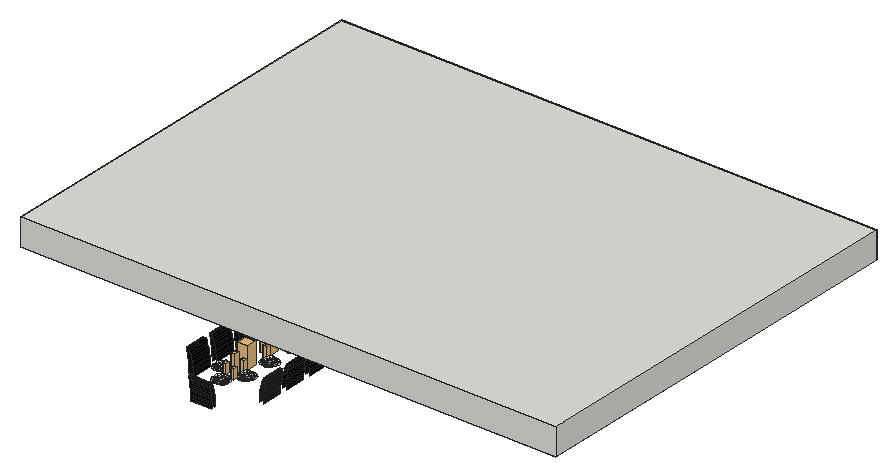
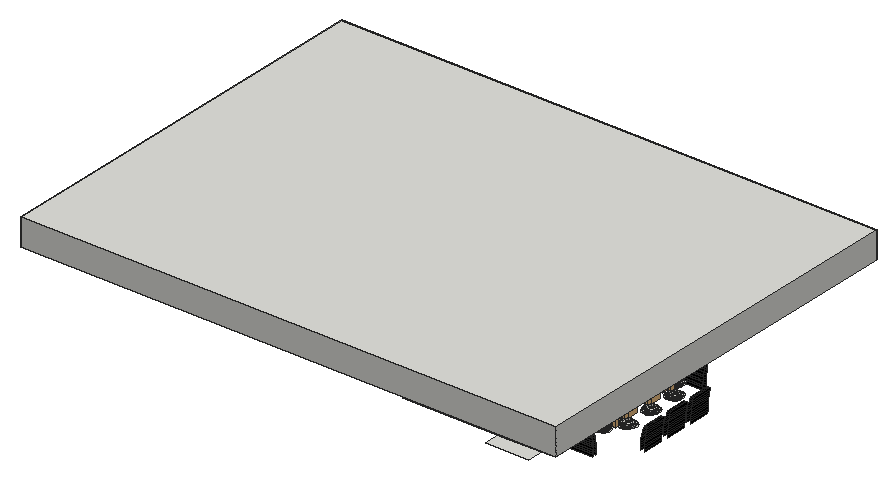
# SketchUp Ruby script. Lengths in inches.
U = 1.inch
M = Sketchup.active_model
def pt(a) = Geom::Point3d.new(a.map { |v| v * U })
def face(e, loops, mat)
  f = e.add_face(loops[0].map { |a| pt(a) })
  loops[1..].each { |l| e.add_face(l.map { |a| pt(a) }).erase! }
  f.material = f.back_material = mat if mat
  f
end
# faces: each face lists its corners as indices into pts; further lists are holes
def faces(e, pts, list, mat = nil) = list.each { |f| face(e, (f[0].is_a?(Array) ? f : [f]).map { |l| l.map { |i| pts[i] } }, mat) }
# xy, xz, yz: faces in a plane at the given z, y or x. An outline is a flat list of corners, or four numbers for a rectangle; further outlines are holes
def ring(l) = l.size == 4 ? [[l[0], l[1]], [l[2], l[1]], [l[2], l[3]], [l[0], l[3]]] : l.each_slice(2).to_a
def flat(e, list, mat, &to3) = list.each { |f| face(e, (f[0].is_a?(Array) ? f : [f]).map { |l| ring(l).map { |u, v| to3.(u, v) } }, mat) }
def xy(e, z, list, mat = nil) = flat(e, list, mat) { |x, y| [x, y, z] }
def xz(e, y, list, mat = nil) = flat(e, list, mat) { |x, z| [x, y, z] }
def yz(e, x, list, mat = nil) = flat(e, list, mat) { |y, z| [x, y, z] }
def lines(e, pts, list) = list.each { |a, b| e.add_line(pt(pts[a]), pt(pts[b])) }
# prism: a flat outline (further loops are holes) pulled along v
def prism(e, loops, v, mat = nil)
  f = face(e, loops, mat); d = Geom::Vector3d.new(v.map { |x| x * U })
  f.pushpull(f.normal.samedirection?(d) ? d.length : -d.length)
end
def box(e, o, s, mat = nil) = prism(e, [[o, [o[0] + s[0], o[1], o[2]], [o[0] + s[0], o[1] + s[1], o[2]], [o[0], o[1] + s[1], o[2]]]], [0, 0, s[2]], mat)
def at(x, y, z, deg = 0) = Geom::Transformation.translation(pt([x, y, z])) * Geom::Transformation.rotation(ORIGIN, Z_AXIS, deg.degrees)
def axes(o, x, y, z) = Geom::Transformation.new([*x, 0, *y, 0, *z, 0, *pt(o).to_a, 1])
def part(name) = M.definitions.add(name)
# library, detail: a bought-in or finely detailed component or shape, given as its bounding box
def library(name, o, s) = part(name).tap { |d| box(d.entities, o, s) }
def detail(e, o, s) = box(e.add_group.entities, o, s)
def put(e, d, t, mat = nil) = e.add_instance(d, t).tap { |i| i.material = mat if mat }
def group(e, t, mat = nil) = e.add_group.tap { |g| g.transformation = t; g.material = mat if mat }.entities
root = M.entities
M.materials.add("[Color M08]").color = [30, 30, 30]
M.materials.add("[Color M09]").color = [0, 0, 0]
c1 = library("Vase with flowers",[0,-0.1,-0.41],[9.125,9.13,19.39])
c2 = library("Candlestick with candle",[0,0,0],[3.93,3.74,15.76])
c3 = library("ske3",[12.02,0,0.58],[3.05,3.06,6.89])
c4 = part("Dishes_Bowl_5in\#1")
xy(c4.entities,0.125,[[-0.25,-0.91,-0.67,-0.67,-0.91,-0.25,-0.91,0.25,-0.67,0.67,-0.25,0.91,0.25,0.91,0.67,0.67,0.91,0.25,0.91,-0.25,0.67,-0.67,0.25,-0.91]])
p = [[-1.16,-1.16,0.41],[-0.67,-0.67,0.125],[-0.25,-0.91,0.125],[-0.43,-1.59,0.41],[0.25,-0.91,0.125],[0.43,-1.59,0.41],
  [0.67,-0.67,0.125],[1.16,-1.16,0.41],[-1.59,-0.43,0.41],[-0.91,-0.25,0.125],[0.91,-0.25,0.125],[1.59,-0.43,0.41],
  [-1.59,0.43,0.41],[-0.91,0.25,0.125],[1.59,0.43,0.41],[0.91,0.25,0.125],[-1.16,1.16,0.41],[-0.67,0.67,0.125],
  [0.67,0.67,0.125],[1.16,1.16,0.41],[-0.43,1.59,0.41],[-0.25,0.91,0.125],[0.25,0.91,0.125],[0.43,1.59,0.41],
  [-1.55,-1.55,0.9375],[-0.57,-2.11,0.9375],[0.57,-2.11,0.9375],[1.55,-1.55,0.9375],[-2.11,-0.57,0.9375],[2.11,-0.57,0.9375],
  [-2.11,0.57,0.9375],[2.11,0.57,0.9375],[-1.55,1.55,0.9375],[1.55,1.55,0.9375],[-0.57,2.11,0.9375],[0.57,2.11,0.9375],
  [-1.77,-1.77,1.625],[-0.65,-2.41,1.625],[0.65,-2.41,1.625],[1.77,-1.77,1.625],[-2.41,-0.65,1.625],[2.41,-0.65,1.625],
  [-2.41,0.65,1.625],[2.41,0.65,1.625],[-1.77,1.77,1.625],[1.77,1.77,1.625],[-0.65,2.41,1.625],[0.65,2.41,1.625]]
faces(c4.entities,p,[[0,1,2,3],[4,5,3,2],[5,4,6,7],[8,9,1,0],[7,6,10,11],[9,8,12,13],[14,11,10,15],[16,17,13,12],
  [14,15,18,19],[20,21,17,16],[19,18,22,23],[20,23,22,21],[24,0,3,25],[5,26,25,3],[26,5,7,27],[28,8,0,24],
  [27,7,11,29],[12,8,28,30],[29,11,14,31],[32,16,12,30],[31,14,19,33],[34,20,16,32],[33,19,23,35],[35,23,20,34],
  [36,24,25,37],[25,26,38,37],[38,26,27,39],[40,28,24,36],[39,27,29,41],[28,40,42,30],[41,29,31,43],[44,32,30,42],
  [43,31,33,45],[46,34,32,44],[45,33,35,47],[47,35,34,46]])
c5 = part("Dishes_Plate_12in\#3")
xy(c5.entities,0.12,[[-0.99,-5,-2.83,-4.24,-4.24,-2.83,-5,-0.99,-5,0.99,-4.24,2.83,-2.83,4.24,-0.99,5,0.99,5,2.83,4.24,4.24,2.83,5,0.99,5,-0.99,4.24,-2.83,2.83,-4.24,0.99,-5]])
xy(c5.entities,0.38,[[[-1.2,-6.02,-3.41,-5.1,-5.1,-3.41,-6.02,-1.2,-6.02,1.2,-5.1,3.41,-3.41,5.1,-1.2,6.02,1.2,6.02,3.41,5.1,5.1,3.41,6.02,1.2,6.02,-1.2,5.1,-3.41,3.41,-5.1,1.2,-6.02],[-0.99,-5,0.99,-5,2.83,-4.24,4.24,-2.83,5,-0.99,5,0.99,4.24,2.83,2.83,4.24,0.99,5,-0.99,5,-2.83,4.24,-4.24,2.83,-5,0.99,-5,-0.99,-4.24,-2.83,-2.83,-4.24]]])
xz(c5.entities,-5,[[-0.99,0.12,0.99,0.38]])
xz(c5.entities,5,[[-0.99,0.12,0.99,0.38]])
yz(c5.entities,-5,[[-0.99,0.12,0.99,0.38]])
yz(c5.entities,5,[[-0.99,0.12,0.99,0.38]])
p = [[-2.83,-4.24,0.12],[-0.99,-5,0.12],[-0.99,-5,0.38],[-2.83,-4.24,0.38],[0.99,-5,0.12],[2.83,-4.24,0.12],
  [2.83,-4.24,0.38],[0.99,-5,0.38],[-4.24,-2.83,0.12],[-4.24,-2.83,0.38],[4.24,-2.83,0.12],[4.24,-2.83,0.38],
  [-5,-0.99,0.12],[-5,-0.99,0.38],[5,-0.99,0.12],[5,-0.99,0.38],[-4.24,2.83,0.12],[-5,0.99,0.12],
  [-5,0.99,0.38],[-4.24,2.83,0.38],[5,0.99,0.12],[4.24,2.83,0.12],[4.24,2.83,0.38],[5,0.99,0.38],
  [-2.83,4.24,0.12],[-2.83,4.24,0.38],[2.83,4.24,0.12],[2.83,4.24,0.38],[-0.99,5,0.12],[-0.99,5,0.38],
  [0.99,5,0.12],[0.99,5,0.38]]
faces(c5.entities,p,[[0,1,2,3],[4,5,6,7],[8,0,3,9],[5,10,11,6],[12,8,9,13],[10,14,15,11],[16,17,18,19],[20,21,22,23],
  [24,16,19,25],[21,26,27,22],[28,24,25,29],[26,30,31,27]])
c6 = part("Dishes_Plate_12in\#4")
xy(c6.entities,0.12,[[-0.99,-5,-2.83,-4.24,-4.24,-2.83,-5,-0.99,-5,0.99,-4.24,2.83,-2.83,4.24,-0.99,5,0.99,5,2.83,4.24,4.24,2.83,5,0.99,5,-0.99,4.24,-2.83,2.83,-4.24,0.99,-5]])
xy(c6.entities,0.38,[[[-1.2,-6.02,-3.41,-5.1,-5.1,-3.41,-6.02,-1.2,-6.02,1.2,-5.1,3.41,-3.41,5.1,-1.2,6.02,1.2,6.02,3.41,5.1,5.1,3.41,6.02,1.2,6.02,-1.2,5.1,-3.41,3.41,-5.1,1.2,-6.02],[-0.99,-5,0.99,-5,2.83,-4.24,4.24,-2.83,5,-0.99,5,0.99,4.24,2.83,2.83,4.24,0.99,5,-0.99,5,-2.83,4.24,-4.24,2.83,-5,0.99,-5,-0.99,-4.24,-2.83,-2.83,-4.24]]])
xz(c6.entities,-5,[[-0.99,0.12,0.99,0.38]])
xz(c6.entities,5,[[-0.99,0.12,0.99,0.38]])
yz(c6.entities,-5,[[-0.99,0.12,0.99,0.38]])
yz(c6.entities,5,[[-0.99,0.12,0.99,0.38]])
p = [[-2.83,-4.24,0.12],[-0.99,-5,0.12],[-0.99,-5,0.38],[-2.83,-4.24,0.38],[0.99,-5,0.12],[2.83,-4.24,0.12],
  [2.83,-4.24,0.38],[0.99,-5,0.38],[-4.24,-2.83,0.12],[-4.24,-2.83,0.38],[4.24,-2.83,0.12],[4.24,-2.83,0.38],
  [-5,-0.99,0.12],[-5,-0.99,0.38],[5,-0.99,0.12],[5,-0.99,0.38],[-4.24,2.83,0.12],[-5,0.99,0.12],
  [-5,0.99,0.38],[-4.24,2.83,0.38],[5,0.99,0.12],[4.24,2.83,0.12],[4.24,2.83,0.38],[5,0.99,0.38],
  [-2.83,4.24,0.12],[-2.83,4.24,0.38],[2.83,4.24,0.12],[2.83,4.24,0.38],[-0.99,5,0.12],[-0.99,5,0.38],
  [0.99,5,0.12],[0.99,5,0.38]]
faces(c6.entities,p,[[0,1,2,3],[4,5,6,7],[8,0,3,9],[5,10,11,6],[12,8,9,13],[10,14,15,11],[16,17,18,19],[20,21,22,23],
  [24,16,19,25],[21,26,27,22],[28,24,25,29],[26,30,31,27]])
c7 = part("Dinnerware place setting")
put(c7.entities,c4,axes([6.08,5.97,0.12],[1.725,0,0],[0,1.725,0],[0,0,1.104]))
put(c7.entities,c5,axes([6.0625,5.99,-0.16],[0.8652,0,0],[0,0.8652,0],[0,0,2.21491]))
put(c7.entities,c6,axes([6.1,6.1,-0.125],[1.01228,0,0],[0,1.01228,0],[0,0,1.01228]))
xy(root,52.03,[[147.72,88.19,150.17,97.38],[147.72,97.38,150.17,106.57]],"[Color M08]")
xy(root,52.03,[[105.17,57.53,114.36,59.98],[114.36,57.53,123.55,59.98],[78.55,88.19,81,97.38],[78.55,97.38,81,106.57],[78.55,114.1,81,123.29],
  [147.72,114.1,150.17,123.29],[78.55,123.29,81,132.48],[147.72,123.29,150.17,132.48],[78.55,140,81,149.19],[147.72,140,150.17,149.19],
  [78.55,149.19,81,158.38],[147.72,149.19,150.17,158.38],[105.17,186.59,114.36,189.04],[114.36,186.59,123.55,189.04]],"[Color M09]")
xy(root,90,[[72,240,110.625,300]])
xy(root,126,[[24,174,60,240],[60,240,156,336]])
xy(root,144,[[0,0,0,360,24,360,24,336,60,336,60,156,24,156,24,0],[24,0,24,156,60,156,60,336,456,336,456,360,480,360,480,0],[24,336,456,360]])
xy(root,168,[[0,0,480,360]])
xz(root,0,[[0,144,480,168]])
xz(root,336,[[24,126,60,144]])
xz(root,360,[[0,144,480,168]])
yz(root,0,[[0,144,360,168]])
yz(root,480,[[0,144,360,168]])
p = [[105.17,60.06,30.79],[105.17,60,32.74],[123.55,60,32.74],[123.55,60.06,30.79],[105.17,63.81,32.79],[105.17,63.75,30.82],
  [123.55,63.75,30.82],[123.55,63.81,32.79],[81.08,106.57,30.79],[81.02,106.57,32.74],[81.02,88.19,32.74],[81.08,88.19,30.79],
  [84.83,106.57,32.79],[84.77,106.57,30.82],[84.77,88.19,30.82],[84.83,88.19,32.79],[143.9,88.19,32.79],[143.95,88.19,30.82],
  [143.95,106.57,30.82],[143.9,106.57,32.79],[147.64,88.19,30.79],[147.7,88.19,32.74],[147.7,106.57,32.74],[147.64,106.57,30.79],
  [81.08,132.48,30.79],[81.02,132.48,32.74],[81.02,114.1,32.74],[81.08,114.1,30.79],[84.83,132.48,32.79],[84.77,132.48,30.82],
  [84.77,114.1,30.82],[84.83,114.1,32.79],[143.9,114.1,32.79],[143.95,114.1,30.82],[143.95,132.48,30.82],[143.9,132.48,32.79],
  [147.64,114.1,30.79],[147.7,114.1,32.74],[147.7,132.48,32.74],[147.64,132.48,30.79],[81.08,158.38,30.79],[81.02,158.38,32.74],
  [81.02,140,32.74],[81.08,140,30.79],[84.83,158.38,32.79],[84.77,158.38,30.82],[84.77,140,30.82],[84.83,140,32.79],
  [143.9,140,32.79],[143.95,140,30.82],[143.95,158.38,30.82],[143.9,158.38,32.79],[147.64,140,30.79],[147.7,140,32.74],
  [147.7,158.38,32.74],[147.64,158.38,30.79],[123.55,182.77,32.79],[123.55,182.82,30.82],[105.17,182.82,30.82],[105.17,182.77,32.79],
  [123.55,186.52,30.79],[123.55,186.58,32.74],[105.17,186.58,32.74],[105.17,186.52,30.79],[105.17,59.91,34.68],[123.55,59.91,34.68],
  [80.92,106.57,34.68],[80.92,88.19,34.68],[147.8,88.19,34.68],[147.8,106.57,34.68],[80.92,132.48,34.68],[80.92,114.1,34.68],
  [147.8,114.1,34.68],[147.8,132.48,34.68],[80.92,158.38,34.68],[80.92,140,34.68],[147.8,140,34.68],[147.8,158.38,34.68],
  [123.55,186.67,34.68],[105.17,186.67,34.68],[105.17,63.78,34.76],[123.55,63.78,34.76],[84.8,106.57,34.76],[84.8,88.19,34.76],
  [143.93,88.19,34.76],[143.93,106.57,34.76],[84.8,132.48,34.76],[84.8,114.1,34.76],[143.93,114.1,34.76],[143.93,132.48,34.76],
  [84.8,158.38,34.76],[84.8,140,34.76],[143.93,140,34.76],[143.93,158.38,34.76],[123.55,182.8,34.76],[105.17,182.8,34.76],
  [105.17,59.78,36.625],[123.55,59.78,36.625],[80.8,106.57,36.625],[80.8,88.19,36.625],[147.93,88.19,36.625],[147.93,106.57,36.625],
  [80.8,132.48,36.625],[80.8,114.1,36.625],[147.93,114.1,36.625],[147.93,132.48,36.625],[80.8,158.38,36.625],[80.8,140,36.625],
  [147.93,140,36.625],[147.93,158.38,36.625],[123.55,186.8,36.625],[105.17,186.8,36.625],[105.17,63.67,36.74],[123.55,63.67,36.74],
  [84.6875,106.57,36.74],[84.6875,88.19,36.74],[144.03,88.19,36.74],[144.03,106.57,36.74],[84.6875,132.48,36.74],[84.6875,114.1,36.74],
  [144.03,114.1,36.74],[144.03,132.48,36.74],[84.6875,158.38,36.74],[84.6875,140,36.74],[144.03,140,36.74],[144.03,158.38,36.74],
  [123.55,182.91,36.74],[105.17,182.91,36.74],[105.17,59.61,38.57],[123.55,59.61,38.57],[80.63,106.57,38.57],[80.63,88.19,38.57],
  [148.09,88.19,38.57],[148.09,106.57,38.57],[80.63,132.48,38.57],[80.63,114.1,38.57],[148.09,114.1,38.57],[148.09,132.48,38.57],
  [80.63,158.38,38.57],[80.63,140,38.57],[148.09,140,38.57],[148.09,158.38,38.57],[123.55,186.96,38.57],[105.17,186.96,38.57],
  [105.17,63.48,38.7],[123.55,63.48,38.7],[84.5,106.57,38.7],[84.5,88.19,38.7],[144.22,88.19,38.7],[144.22,106.57,38.7],
  [84.5,132.48,38.7],[84.5,114.1,38.7],[144.22,114.1,38.7],[144.22,132.48,38.7],[84.5,158.38,38.7],[84.5,140,38.7],
  [144.22,140,38.7],[144.22,158.38,38.7],[123.55,183.09,38.7],[105.17,183.09,38.7],[105.17,59.42,40.5],[123.55,59.42,40.5],
  [80.4375,106.57,40.5],[80.4375,88.19,40.5],[148.29,88.19,40.5],[148.29,106.57,40.5],[80.4375,132.48,40.5],[80.4375,114.1,40.5],
  [148.29,114.1,40.5],[148.29,132.48,40.5],[80.4375,158.38,40.5],[80.4375,140,40.5],[148.29,140,40.5],[148.29,158.38,40.5],
  [123.55,187.16,40.5],[105.17,187.16,40.5],[105.17,63.22,40.66],[123.55,63.22,40.66],[84.24,106.57,40.66],[84.24,88.19,40.66],
  [144.49,88.19,40.66],[144.49,106.57,40.66],[84.24,132.48,40.66],[84.24,114.1,40.66],[144.49,114.1,40.66],[144.49,132.48,40.66],
  [84.24,158.38,40.66],[84.24,140,40.66],[144.49,140,40.66],[144.49,158.38,40.66],[123.55,183.36,40.66],[105.17,183.36,40.66],
  [105.17,59.1875,42.4375],[123.55,59.1875,42.4375],[80.21,106.57,42.4375],[80.21,88.19,42.4375],[148.52,88.19,42.4375],[148.52,106.57,42.4375],
  [80.21,132.48,42.4375],[80.21,114.1,42.4375],[148.52,114.1,42.4375],[148.52,132.48,42.4375],[80.21,158.38,42.4375],[80.21,140,42.4375],
  [148.52,140,42.4375],[148.52,158.38,42.4375],[123.55,187.39,42.4375],[105.17,187.39,42.4375],[105.17,62.87,42.6],[123.55,62.87,42.6],
  [83.89,106.57,42.6],[83.89,88.19,42.6],[144.83,88.19,42.6],[144.83,106.57,42.6],[83.89,132.48,42.6],[83.89,114.1,42.6],
  [144.83,114.1,42.6],[144.83,132.48,42.6],[83.89,158.38,42.6],[83.89,140,42.6],[144.83,140,42.6],[144.83,158.38,42.6],
  [123.55,183.71,42.6],[105.17,183.71,42.6],[105.17,58.93,44.37],[123.55,58.93,44.37],[79.94,106.57,44.37],[79.94,88.19,44.37],
  [148.78,88.19,44.37],[148.78,106.57,44.37],[79.94,132.48,44.37],[79.94,114.1,44.37],[148.78,114.1,44.37],[148.78,132.48,44.37],
  [79.94,158.38,44.37],[79.94,140,44.37],[148.78,140,44.37],[148.78,158.38,44.37],[123.55,187.65,44.37],[105.17,187.65,44.37],
  [105.17,62.45,44.53],[123.55,62.45,44.53],[83.47,106.57,44.53],[83.47,88.19,44.53],[145.26,88.19,44.53],[145.26,106.57,44.53],
  [83.47,132.48,44.53],[83.47,114.1,44.53],[145.26,114.1,44.53],[145.26,132.48,44.53],[83.47,158.38,44.53],[83.47,140,44.53],
  [145.26,140,44.53],[145.26,158.38,44.53],[123.55,184.13,44.53],[105.17,184.13,44.53],[105.17,58.63,46.29],[123.55,58.63,46.29],
  [79.65,106.57,46.29],[79.65,88.19,46.29],[149.08,88.19,46.29],[149.08,106.57,46.29],[79.65,132.48,46.29],[79.65,114.1,46.29],
  [149.08,114.1,46.29],[149.08,132.48,46.29],[79.65,158.38,46.29],[79.65,140,46.29],[149.08,140,46.29],[149.08,158.38,46.29],
  [123.55,187.95,46.29],[105.17,187.95,46.29],[105.17,61.95,46.44],[123.55,61.95,46.44],[82.96,106.57,46.44],[82.96,88.19,46.44],
  [145.76,88.19,46.44],[145.76,106.57,46.44],[82.96,132.48,46.44],[82.96,114.1,46.44],[145.76,114.1,46.44],[145.76,132.48,46.44],
  [82.96,158.38,46.44],[82.96,140,46.44],[145.76,140,46.44],[145.76,158.38,46.44],[123.55,184.63,46.44],[105.17,184.63,46.44],
  [105.17,58.3,48.21],[123.55,58.3,48.21],[79.32,106.57,48.21],[79.32,88.19,48.21],[149.41,88.19,48.21],[149.41,106.57,48.21],
  [79.32,132.48,48.21],[79.32,114.1,48.21],[149.41,114.1,48.21],[149.41,132.48,48.21],[79.32,158.38,48.21],[79.32,140,48.21],
  [149.41,140,48.21],[149.41,158.38,48.21],[123.55,188.28,48.21],[105.17,188.28,48.21],[105.17,61.37,48.33],[123.55,61.37,48.33],
  [82.39,106.57,48.33],[82.39,88.19,48.33],[146.34,88.19,48.33],[146.34,106.57,48.33],[82.39,132.48,48.33],[82.39,114.1,48.33],
  [146.34,114.1,48.33],[146.34,132.48,48.33],[82.39,158.38,48.33],[82.39,140,48.33],[146.34,140,48.33],[146.34,158.38,48.33],
  [123.55,185.21,48.33],[105.17,185.21,48.33],[105.17,57.93,50.12],[123.55,57.93,50.12],[78.95,106.57,50.12],[78.95,88.19,50.12],
  [149.77,88.19,50.12],[149.77,106.57,50.12],[78.95,132.48,50.12],[78.95,114.1,50.12],[149.77,114.1,50.12],[149.77,132.48,50.12],
  [78.95,158.38,50.12],[78.95,140,50.12],[149.77,140,50.12],[149.77,158.38,50.12],[123.55,188.64,50.12],[105.17,188.64,50.12],
  [105.17,60.71,50.19],[123.55,60.71,50.19],[114.36,60.71,50.19],[81.73,106.57,50.19],[81.73,88.19,50.19],[81.73,97.38,50.19],
  [146.99,88.19,50.19],[146.99,106.57,50.19],[146.99,97.38,50.19],[81.73,132.48,50.19],[81.73,114.1,50.19],[81.73,123.29,50.19],
  [146.99,114.1,50.19],[146.99,132.48,50.19],[146.99,123.29,50.19],[81.73,158.38,50.19],[81.73,140,50.19],[81.73,149.19,50.19],
  [146.99,140,50.19],[146.99,158.38,50.19],[146.99,149.19,50.19],[123.55,185.86,50.19],[105.17,185.86,50.19],[114.36,185.86,50.19],
  [105.17,57.53,52.03],[114.36,57.53,52.03],[123.55,57.53,52.03],[78.55,106.57,52.03],[78.55,97.38,52.03],[78.55,88.19,52.03],
  [150.17,88.19,52.03],[150.17,97.38,52.03],[150.17,106.57,52.03],[78.55,132.48,52.03],[78.55,123.29,52.03],[78.55,114.1,52.03],
  [150.17,114.1,52.03],[150.17,123.29,52.03],[150.17,132.48,52.03],[78.55,158.38,52.03],[78.55,149.19,52.03],[78.55,140,52.03],
  [150.17,140,52.03],[150.17,149.19,52.03],[150.17,158.38,52.03],[123.55,189.04,52.03],[114.36,189.04,52.03],[105.17,189.04,52.03],
  [105.17,59.98,52.03],[114.36,59.98,52.03],[123.55,59.98,52.03],[81,88.19,52.03],[81,97.38,52.03],[147.72,88.19,52.03],
  [147.72,97.38,52.03],[81,106.57,52.03],[147.72,106.57,52.03],[81,114.1,52.03],[81,123.29,52.03],[147.72,114.1,52.03],
  [147.72,123.29,52.03],[81,132.48,52.03],[147.72,132.48,52.03],[81,140,52.03],[81,149.19,52.03],[147.72,140,52.03],
  [147.72,149.19,52.03],[81,158.38,52.03],[147.72,158.38,52.03],[105.17,186.59,52.03],[114.36,186.59,52.03],[123.55,186.59,52.03]]
faces(root,p,[[0,1,2,3],[4,5,6,7],[8,9,10,11],[12,13,14,15],[24,25,26,27],[28,29,30,31],[32,33,34,35],[36,37,38,39],
  [40,41,42,43],[44,45,46,47],[48,49,50,51],[52,53,54,55],[56,57,58,59],[60,61,62,63],[1,64,65,2],[9,66,67,10],
  [25,70,71,26],[37,72,73,38],[41,74,75,42],[53,76,77,54],[61,78,79,62],[80,4,7,81],[82,12,15,83],[86,28,31,87],
  [88,32,35,89],[90,44,47,91],[92,48,51,93],[94,56,59,95],[64,96,97,65],[66,98,99,67],[70,102,103,71],[72,104,105,73],
  [74,106,107,75],[76,108,109,77],[78,110,111,79],[112,80,81,113],[114,82,83,115],[118,86,87,119],[120,88,89,121],[122,90,91,123],
  [124,92,93,125],[126,94,95,127],[96,128,129,97],[98,130,131,99],[102,134,135,103],[104,136,137,105],[106,138,139,107],[108,140,141,109],
  [110,142,143,111],[144,112,113,145],[146,114,115,147],[150,118,119,151],[152,120,121,153],[154,122,123,155],[156,124,125,157],[158,126,127,159],
  [128,160,161,129],[130,162,163,131],[134,166,167,135],[136,168,169,137],[138,170,171,139],[140,172,173,141],[142,174,175,143],[176,144,145,177],
  [178,146,147,179],[182,150,151,183],[184,152,153,185],[186,154,155,187],[188,156,157,189],[190,158,159,191],[160,192,193,161],[162,194,195,163],
  [166,198,199,167],[168,200,201,169],[170,202,203,171],[172,204,205,173],[174,206,207,175],[208,176,177,209],[210,178,179,211],[214,182,183,215],
  [216,184,185,217],[218,186,187,219],[220,188,189,221],[222,190,191,223],[192,224,225,193],[194,226,227,195],[198,230,231,199],[200,232,233,201],
  [202,234,235,203],[204,236,237,205],[206,238,239,207],[240,208,209,241],[242,210,211,243],[246,214,215,247],[248,216,217,249],[250,218,219,251],
  [252,220,221,253],[254,222,223,255],[224,256,257,225],[226,258,259,227],[230,262,263,231],[232,264,265,233],[234,266,267,235],[236,268,269,237],
  [238,270,271,239],[272,240,241,273],[274,242,243,275],[278,246,247,279],[280,248,249,281],[282,250,251,283],[284,252,253,285],[286,254,255,287],
  [256,288,289,257],[258,290,291,259],[262,294,295,263],[264,296,297,265],[266,298,299,267],[268,300,301,269],[270,302,303,271],[304,272,273,305],
  [306,274,275,307],[310,278,279,311],[312,280,281,313],[314,282,283,315],[316,284,285,317],[318,286,287,319],[288,320,321,289],[290,322,323,291],
  [294,326,327,295],[296,328,329,297],[298,330,331,299],[300,332,333,301],[302,334,335,303],[336,304,305,337,338],[339,306,307,340,341],[345,310,311,346,347],
  [348,312,313,349,350],[351,314,315,352,353],[354,316,317,355,356],[357,318,319,358,359],[360,361,362,321,320],[363,364,365,323,322],[369,370,371,327,326],[372,373,374,329,328],
  [375,376,377,331,330],[378,379,380,333,332],[381,382,383,335,334],[384,336,338,385],[337,386,385,338],[340,387,388,341],[391,339,341,388],[346,393,394,347],
  [395,348,350,396],[397,345,347,394],[349,398,396,350],[352,399,400,353],[401,354,356,402],[403,351,353,400],[355,404,402,356],[358,405,406,359],
  [407,357,359,406]],"[Color M09]")
faces(root,p,[[16,17,18,19],[20,21,22,23],[21,68,69,22],[84,16,19,85],[68,100,101,69],[116,84,85,117],[100,132,133,101],[148,116,117,149],
  [132,164,165,133],[180,148,149,181],[164,196,197,165],[212,180,181,213],[196,228,229,197],[244,212,213,245],[228,260,261,229],[276,244,245,277],
  [260,292,293,261],[308,276,277,309],[292,324,325,293],[342,308,309,343,344],[366,367,368,325,324],[389,342,344,390],[343,392,390,344]],"[Color M08]")
put(root,c1,at(109.85,105.98,40.82))
put(root,c1,at(118.875,140.6,40.82,180))
put(root,c2,at(116.33,151.22,40.85,180))
put(root,c2,at(112.4,95.36,40.85))
put(root,c3,axes([125.6,145.5,40.12],[-1.1,0,0],[0,-1.1,0],[0,0,1.32]))
put(root,c3,axes([103.12,152.89,40.12],[1.1,0,0],[0,1.1,0],[0,0,1.32]))
put(root,c3,axes([103.12,101.08,40.12],[1.1,0,0],[0,1.1,0],[0,0,1.32]))
put(root,c3,axes([125.6,93.6875,40.12],[-1.1,0,0],[0,-1.1,0],[0,0,1.32]))
put(root,c3,axes([118.06,104.58,40.12],[0,-1.1,0],[1.1,0,0],[0,0,1.32]))
put(root,c3,axes([103.12,126.98,40.12],[1.1,0,0],[0,1.1,0],[0,0,1.32]))
put(root,c3,axes([110.67,142,40.12],[0,1.1,0],[-1.1,0,0],[0,0,1.32]))
put(root,c3,axes([125.6,119.59,40.12],[-1.1,0,0],[0,-1.1,0],[0,0,1.32]))
put(root,c7,axes([96.12,104.69,40.93],[0,-1.199,0],[1.199,0,0],[0,0,1.199]))
put(root,c7,axes([96.12,156.5,40.93],[0,-1.199,0],[1.199,0,0],[0,0,1.199]))
put(root,c7,axes([132.6,90.07,40.93],[0,1.199,0],[-1.199,0,0],[0,0,1.199]))
put(root,c7,axes([132.6,141.89,40.93],[0,1.199,0],[-1.199,0,0],[0,0,1.199]))
put(root,c7,axes([121.67,171.48,40.93],[-1.199,0,0],[0,-1.199,0],[0,0,1.199]))
put(root,c7,axes([96.12,130.6,40.93],[0,-1.199,0],[1.199,0,0],[0,0,1.199]))
put(root,c7,axes([107.05,75.1,40.93],[1.199,0,0],[0,1.199,0],[0,0,1.199]))
put(root,c7,axes([132.6,115.98,40.93],[0,1.199,0],[-1.199,0,0],[0,0,1.199]))
